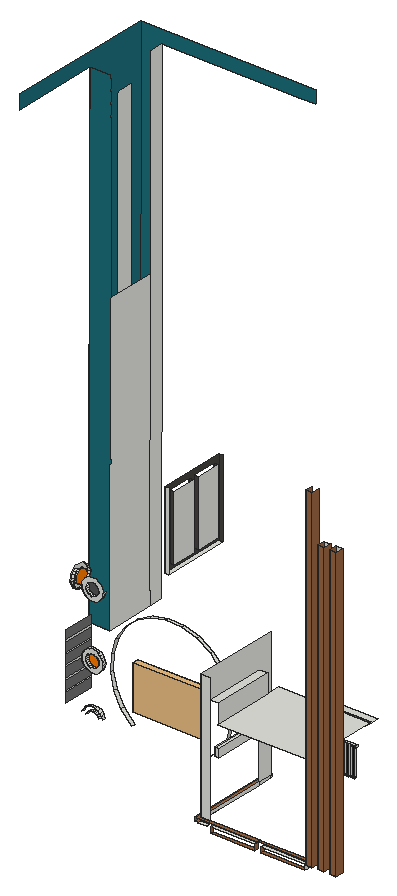
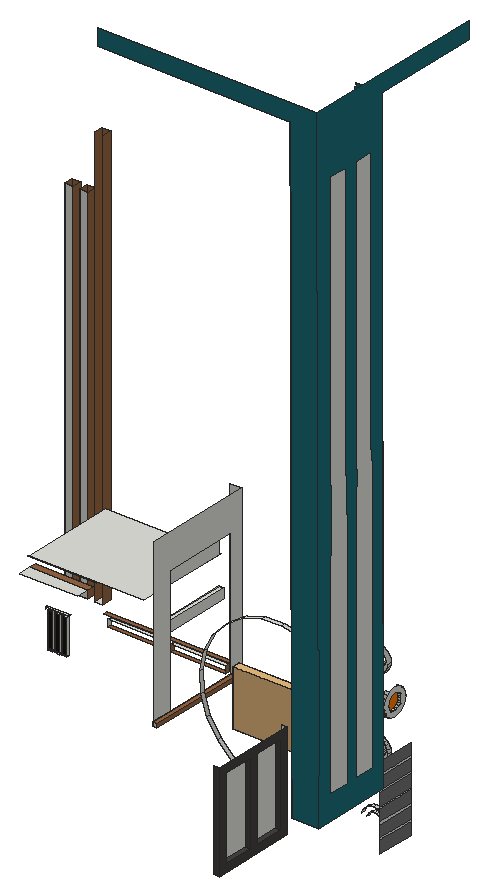
# SketchUp Ruby script. Lengths in inches.
U = 1.inch
M = Sketchup.active_model
def pt(a) = Geom::Point3d.new(a.map { |v| v * U })
def face(e, loops, mat)
  f = e.add_face(loops[0].map { |a| pt(a) })
  loops[1..].each { |l| e.add_face(l.map { |a| pt(a) }).erase! }
  f.material = f.back_material = mat if mat
  f
end
# faces: each face lists its corners as indices into pts; further lists are holes
def faces(e, pts, list, mat = nil) = list.each { |f| face(e, (f[0].is_a?(Array) ? f : [f]).map { |l| l.map { |i| pts[i] } }, mat) }
# xy, xz, yz: faces in a plane at the given z, y or x. An outline is a flat list of corners, or four numbers for a rectangle; further outlines are holes
def ring(l) = l.size == 4 ? [[l[0], l[1]], [l[2], l[1]], [l[2], l[3]], [l[0], l[3]]] : l.each_slice(2).to_a
def flat(e, list, mat, &to3) = list.each { |f| face(e, (f[0].is_a?(Array) ? f : [f]).map { |l| ring(l).map { |u, v| to3.(u, v) } }, mat) }
def xy(e, z, list, mat = nil) = flat(e, list, mat) { |x, y| [x, y, z] }
def xz(e, y, list, mat = nil) = flat(e, list, mat) { |x, z| [x, y, z] }
def yz(e, x, list, mat = nil) = flat(e, list, mat) { |y, z| [x, y, z] }
def lines(e, pts, list) = list.each { |a, b| e.add_line(pt(pts[a]), pt(pts[b])) }
# prism: a flat outline (further loops are holes) pulled along v
def prism(e, loops, v, mat = nil)
  f = face(e, loops, mat); d = Geom::Vector3d.new(v.map { |x| x * U })
  f.pushpull(f.normal.samedirection?(d) ? d.length : -d.length)
end
def box(e, o, s, mat = nil) = prism(e, [[o, [o[0] + s[0], o[1], o[2]], [o[0] + s[0], o[1] + s[1], o[2]], [o[0], o[1] + s[1], o[2]]]], [0, 0, s[2]], mat)
def at(x, y, z, deg = 0) = Geom::Transformation.translation(pt([x, y, z])) * Geom::Transformation.rotation(ORIGIN, Z_AXIS, deg.degrees)
def axes(o, x, y, z) = Geom::Transformation.new([*x, 0, *y, 0, *z, 0, *pt(o).to_a, 1])
def part(name) = M.definitions.add(name)
# library, detail: a bought-in or finely detailed component or shape, given as its bounding box
def library(name, o, s) = part(name).tap { |d| box(d.entities, o, s) }
def detail(e, o, s) = box(e.add_group.entities, o, s)
def put(e, d, t, mat = nil) = e.add_instance(d, t).tap { |i| i.material = mat if mat }
def group(e, t, mat = nil) = e.add_group.tap { |g| g.transformation = t; g.material = mat if mat }.entities
root = M.entities
M.materials.add("C05_Golden_Blaze").color = [255, 123, 0]
M.materials.add("I06_Sapphire_Night").color = [28, 110, 122]
M.materials.add("M05_Graphite_Haze").color = [114, 114, 114]
M.materials.add("M06_Steel_Smoke").color = [86, 86, 86]
M.materials.add("Wood_Floor_12_1K").color = [28, 22, 19]
M.materials.add("Wood_Planks_01_1K").color = [69, 67, 63]
M.materials.add("Wood_Veneer_15_1K").color = [153, 102, 66]
c1 = library("ALL HOUSE  DESIG",[0.14,0,0],[101.96,32.66,1])
box(root,[157.14,58,93.95],[2.5,40,5.23])
xy(root,54.33,[[161.64,48.875,190.64,50.875],[194.64,48.875,223.64,50.875]],"Wood_Veneer_15_1K")
xy(root,58,[[161.64,48.875,190.64,50.875],[194.64,48.875,223.64,50.875]])
xy(root,58,[[[151.11,48.875,151.11,109.2,153.64,109.2,153.64,50.875,159.64,50.875,159.64,48.875],[151.68,101.68,152.875,103],[151.68,93.68,152.875,95],[151.68,85.6875,152.875,87.01],[151.68,77.69,152.875,79.01],[151.68,69.7,152.875,71.02],[151.68,61.7,152.875,63.02]]],"Wood_Veneer_15_1K")
xy(root,58.02,[[153.64,48,159.64,50.875]])
xy(root,60,[[151.11,48.875,192.14,48.875,192.14,50.875,153.64,50.875,153.64,109.2,151.11,109.2],[193.14,48.875,225.64,50.875]],"Wood_Veneer_15_1K")
xy(root,61.78,[[228.57,43,232.92,48]])
xy(root,61.91,[[236.45,43,240.8,48]])
xy(root,62.04,[[244.33,43,248.68,48]])
xy(root,75.66,[[197.19,109.5,199.99,110.5],[200.99,109.5,203.79,110.5],[204.79,109.5,207.59,110.5]])
xy(root,76.43,[[197.19,109.5,199.99,110.5],[200.99,109.5,203.79,110.5],[204.79,109.5,207.59,110.5]])
xy(root,92.42,[[15.64,193.5,18.64,237.59]])
xy(root,94.34,[[197.19,109.5,199.99,110.5],[200.99,109.5,203.79,110.5],[204.79,109.5,207.59,110.5]])
xy(root,95.34,[[196.19,109.5,208.59,110.5]])
xy(root,96.42,[[15.64,197.5,18.64,213.54],[15.64,217.54,18.64,233.59]],"Wood_Planks_01_1K")
xy(root,111,[[186.64,110.5,216.64,117]])
xy(root,111,[[186.64,107,216.64,110.5]],"Wood_Veneer_15_1K")
xy(root,114,[[159.64,56.88,219.64,107]])
xy(root,114,[[183.64,107,219.64,108]],"Wood_Veneer_15_1K")
xy(root,126,[[[153.64,58,159.64,98],[158.35,92.29,158.94,95.07],[158.35,85.8,158.94,88.58],[158.35,79.31,158.94,82.09],[158.35,72.81,158.94,75.6],[158.35,66.32,158.94,69.11],[158.35,59.83,158.94,62.61]]])
xz(root,43,[[228.57,61.78,232.92,281.97],[236.45,61.91,240.8,252.41],[244.33,62.04,248.68,252.41]],"Wood_Veneer_15_1K")
xz(root,48,[[236.45,61.91,240.8,252.41],[244.33,62.04,248.68,252.41]])
xz(root,50.875,[[153.64,58,159.64,58.02],[153.64,58.02,159.64,60],[153.64,60,159.64,144]])
xz(root,106,[[[38.08,80.04,39.89,80.22,41.6,80.87,43.08,81.93,44.24,83.34,44.99,85,45.29,86.8,45.11,88.62,44.46,90.33,43.4,91.81,41.99,92.96,40.33,93.72,38.53,94.01,36.71,93.83,35,93.1875,33.52,92.125,32.37,90.71,31.61,89.05,31.32,87.25,31.5,85.4375,32.14,83.73,33.21,82.25,34.62,81.09,36.28,80.34],[38.3,82.78,37.2,82.93,36.18,83.35,35.3,84.03,34.625,84.91,34.2,85.93,34.06,87.03,34.2,88.125,34.625,89.15,35.3,90.03,36.18,90.7,37.2,91.13,38.3,91.27,39.4,91.13,40.43,90.7,41.3,90.03,41.98,89.15,42.4,88.125,42.55,87.03,42.4,85.93,41.98,84.91,41.3,84.03,40.43,83.35,39.4,82.93]],[[38.08,122.25,39.89,122.43,41.6,123.07,43.08,124.13,44.24,125.54,44.99,127.21,45.29,129.01,45.11,130.82,44.46,132.53,43.4,134.01,41.99,135.17,40.33,135.92,38.53,136.22,36.71,136.04,35,135.39,33.52,134.33,32.37,132.92,31.61,131.25,31.32,129.45,31.5,127.64,32.14,125.93,33.21,124.45,34.62,123.29,36.28,122.54],[38.17,124.95,37.0625,125.13,36.04,125.59,35.18,126.3,34.53,127.21,34.13,128.26,34.02,129.37,34.2,130.47,34.66,131.49,35.37,132.36,36.28,133.01,37.33,133.4,38.44,133.51,39.54,133.33,40.5625,132.87,41.43,132.16,42.08,131.25,42.47,130.21,42.58,129.09,42.4,127.99,41.94,126.97,41.23,126.11,40.32,125.45,39.28,125.06]]])
xz(root,108,[[38.3,82.78,39.4,82.93,40.43,83.35,41.3,84.03,41.98,84.91,42.4,85.93,42.55,87.03,42.4,88.125,41.98,89.15,41.3,90.03,40.43,90.7,39.4,91.13,38.3,91.27,37.2,91.13,36.18,90.7,35.3,90.03,34.625,89.15,34.2,88.125,34.06,87.03,34.2,85.93,34.625,84.91,35.3,84.03,36.18,83.35,37.2,82.93]],"C05_Golden_Blaze")
xz(root,108,[[38.17,124.95,39.28,125.06,40.32,125.45,41.23,126.11,41.94,126.97,42.4,127.99,42.58,129.09,42.47,130.21,42.08,131.25,41.43,132.16,40.5625,132.87,39.54,133.33,38.44,133.51,37.33,133.4,36.28,133.01,35.37,132.36,34.66,131.49,34.2,130.47,34.02,129.37,34.13,128.26,34.53,127.21,35.18,126.3,36.04,125.59,37.0625,125.13]],"M06_Steel_Smoke")
xz(root,109.2,[[151.11,58,153.64,60]])
xz(root,110.5,[[197.19,76.43,199.99,94.34],[200.99,76.43,203.79,94.34],[204.79,76.43,207.59,94.34]],"Wood_Floor_12_1K")
xz(root,134.17,[[27.27,88.73,27.64,284.16,27.64,284.36,27.82,380.13,27.84,390.13,26.84,390.13,26.84,392.13,27.84,392.13,27.85,397.81,26.85,397.81,26.86,399.81,27.86,399.81,27.87,405.49,26.87,405.49,26.875,407.49,27.875,407.49,27.88,413.16,26.88,413.17,26.89,415.17,13.74,415.19,13.12,88.76]],"I06_Sapphire_Night")
xz(root,176.1875,[[27.27,88.73,13.12,88.76,13.75,424.19,128.6,423.97,128.58,415.15,119.58,415.16,27.89,415.16,27.84,390.13,27.82,380.13,27.64,284.16]],"I06_Sapphire_Night")
xz(root,193.5,[[15.64,92.42,18.64,143.3]])
xz(root,197.5,[[15.64,96.42,18.64,139.3]],"Wood_Planks_01_1K")
xz(root,213.54,[[15.64,96.42,18.64,139.3]],"Wood_Planks_01_1K")
xz(root,217.54,[[15.64,96.42,18.64,139.3]],"Wood_Planks_01_1K")
xz(root,233.59,[[15.64,96.42,18.64,139.3]],"Wood_Planks_01_1K")
xz(root,237.59,[[15.64,92.42,18.64,143.3]],"Wood_Planks_01_1K")
yz(root,15.64,[[[193.5,92.42,237.59,143.3],[217.54,96.42,233.59,139.3],[197.5,96.42,213.54,139.3]]],"Wood_Planks_01_1K")
yz(root,16.64,[[[122.03,116,120.22,116.18,118.51,116.82,117.03,117.89,115.875,119.3,115.12,120.96,114.83,122.76,115.01,124.58,115.65,126.28,116.71,127.76,118.125,128.92,119.79,129.67,121.59,129.97,123.4,129.79,125.11,129.14,126.59,128.08,127.75,126.67,128.5,125.01,128.8,123.21,128.62,121.39,127.97,119.6875,126.91,118.2,125.5,117.05,123.83,116.3],[121.8125,118.74,122.91,118.88,123.93,119.31,124.8125,119.98,125.49,120.86,125.91,121.89,126.06,122.98,125.91,124.08,125.49,125.11,124.8125,125.99,123.93,126.66,122.91,127.08,121.8125,127.23,120.71,127.08,119.6875,126.66,118.81,125.99,118.13,125.11,117.71,124.08,117.57,122.98,117.71,121.89,118.13,120.86,118.81,119.98,119.6875,119.31,120.71,118.88]]])
yz(root,18.64,[[109,60.57,128.87,61.57],[109,68.01,128.87,69.01],[109,75.46,128.87,76.46],[109,82.9,128.87,83.9],[109,90.35,128.87,91.35],
  [197.5,96.42,213.54,139.3],[217.54,96.42,233.59,139.3]])
yz(root,18.64,[[121.8125,118.74,120.71,118.88,119.6875,119.31,118.81,119.98,118.13,120.86,117.71,121.89,117.57,122.98,117.71,124.08,118.13,125.11,118.81,125.99,119.6875,126.66,120.71,127.08,121.8125,127.23,122.91,127.08,123.93,126.66,124.8125,125.99,125.49,125.11,125.91,124.08,126.06,122.98,125.91,121.89,125.49,120.86,124.8125,119.98,123.93,119.31,122.91,118.88]],"C05_Golden_Blaze")
yz(root,18.64,[[109,54.12,128.87,60.57],[109,61.57,128.87,68.01],[109,69.01,128.87,75.46],[109,76.46,128.87,82.9],[109,83.9,128.87,90.35],
  [109,91.35,128.87,97.35]],"M05_Graphite_Haze")
yz(root,151.11,[[48.875,58,109.2,60]],"Wood_Veneer_15_1K")
yz(root,153.64,[[50.875,58,58,60],[58,58,98,60],[98,58,108,60],[108,58,109.2,60],[50.875,60,50.875,144,108,144,108,60,98,60,98,126,58,126,58,60]])
yz(root,159.64,[[48.875,58,50.875,58.02],[58,114,98,126]])
yz(root,161.64,[[48.875,54.33,50.875,58]],"Wood_Veneer_15_1K")
yz(root,190.64,[[48.875,54.33,50.875,58]],"Wood_Veneer_15_1K")
yz(root,194.64,[[48.875,54.33,50.875,58]],"Wood_Veneer_15_1K")
yz(root,197.19,[[109.5,76.43,110.5,94.34]])
yz(root,199.99,[[109.5,76.43,110.5,94.34]])
yz(root,200.99,[[109.5,76.43,110.5,94.34]])
yz(root,203.79,[[109.5,76.43,110.5,94.34]])
yz(root,204.79,[[109.5,76.43,110.5,94.34]])
yz(root,207.59,[[109.5,75.66,110.5,76.43],[109.5,76.43,110.5,94.34]])
yz(root,208.59,[[109.5,94.34,110.5,95.34]])
yz(root,223.64,[[48.875,54.33,50.875,58]])
yz(root,228.57,[[43,61.78,48,281.97]],"Wood_Veneer_15_1K")
yz(root,232.92,[[43,61.78,48,281.97]],"Wood_Veneer_15_1K")
yz(root,236.45,[[43,61.91,48,252.41]],"Wood_Veneer_15_1K")
yz(root,240.8,[[43,61.91,48,252.41]],"Wood_Veneer_15_1K")
yz(root,244.33,[[43,62.04,48,252.41]],"Wood_Veneer_15_1K")
yz(root,248.68,[[43,62.04,48,252.41]],"Wood_Veneer_15_1K")
p = [[34.2,108,54.32],[34.625,108,55.34],[34.625,106,55.34],[34.2,106,54.32],[41.98,108,55.34],[42.4,108,54.32],
  [42.4,106,54.32],[41.98,106,55.34],[45.11,108,54.81],[44.46,108,56.52],[44.46,106,56.52],[45.11,106,54.81],
  [32.37,108,56.9],[31.61,108,55.24],[31.61,106,55.24],[32.37,106,56.9],[35.3,108,56.22],[35.3,106,56.22],
  [41.3,108,56.22],[41.3,106,56.22],[112.8,108,55.62],[120.51,108,62.64],[120.51,106,62.64],[112.8,106,55.62],
  [36.18,108,56.89],[36.18,106,56.89],[40.43,108,56.89],[40.43,106,56.89],[43.4,108,58],[43.4,106,58],
  [33.52,108,58.32],[33.52,106,58.32],[37.2,108,57.32],[37.2,106,57.32],[39.4,108,57.32],[39.4,106,57.32],
  [38.3,108,57.46],[38.3,106,57.46],[57.2,108,65.59],[64.22,108,57.88],[64.22,106,57.88],[57.2,106,65.59],
  [41.99,108,59.15],[41.99,106,59.15],[35,108,59.38],[35,106,59.38],[40.33,108,59.91],[40.33,106,59.91],
  [36.71,108,60.02],[36.71,106,60.02],[38.53,108,60.2],[38.53,106,60.2],[126.14,108,71.42],[126.14,106,71.42],
  [52.42,108,74.86],[52.42,106,74.86],[129.3,108,81.35],[129.3,106,81.35],[50.19,108,85.04],[50.19,106,85.04],
  [36.28,108,80.34],[38.08,108,80.04],[38.08,106,80.04],[36.28,106,80.34],[39.89,108,80.22],[39.89,106,80.22],
  [41.6,108,80.87],[41.6,106,80.87],[34.62,108,81.09],[34.62,106,81.09],[43.08,108,81.93],[43.08,106,81.93],
  [33.21,108,82.25],[33.21,106,82.25],[129.79,108,91.77],[129.79,106,91.77],[44.24,108,83.34],[44.24,106,83.34],
  [32.14,108,83.73],[32.14,106,83.73],[38.3,108,82.78],[37.2,108,82.93],[37.2,106,82.93],[38.3,106,82.78],
  [39.4,108,82.93],[39.4,106,82.93],[36.18,108,83.35],[36.18,106,83.35],[40.43,108,83.35],[40.43,106,83.35],
  [44.99,108,85],[44.99,106,85],[35.3,108,84.03],[35.3,106,84.03],[41.3,108,84.03],[41.3,106,84.03],
  [31.5,108,85.4375],[31.5,106,85.4375],[34.625,108,84.91],[34.625,106,84.91],[41.98,108,84.91],[41.98,106,84.91],
  [34.2,108,85.93],[34.2,106,85.93],[42.4,108,85.93],[42.4,106,85.93],[45.29,108,86.8],[45.29,106,86.8],
  [50.68,108,95.46],[50.68,106,95.46],[31.32,108,87.25],[31.32,106,87.25],[34.06,108,87.03],[34.06,106,87.03],
  [42.55,108,87.03],[42.55,106,87.03],[45.11,108,88.62],[45.11,106,88.62],[34.2,108,88.125],[34.2,106,88.125],
  [42.4,108,88.125],[42.4,106,88.125],[31.61,108,89.05],[31.61,106,89.05],[34.625,108,89.15],[34.625,106,89.15],
  [41.98,108,89.15],[41.98,106,89.15],[44.46,108,90.33],[44.46,106,90.33],[27.27,167.15,88.73],[27.27,134.17,88.73],
  [13.12,134.17,88.76],[13.12,176.1875,88.76],[27.27,176.1875,88.73],[27.64,167.15,284.16],[27.64,134.17,284.16],[27.89,176.1875,415.16],
  [27.89,167.15,415.16],[27.84,167.15,390.13],[27.82,167.15,380.13],[27.64,167.15,284.36],[27.64,176.1875,284.16],[27.82,176.1875,380.13],
  [27.84,176.1875,390.13],[13.75,77.1875,424.19],[13.75,176.1875,424.19],[13.74,134.17,415.19],[13.74,77.1875,415.19],[13.69,157.68,390.5],
  [13.14,157.68,101.81],[13.14,167.91,101.81],[13.69,167.91,390.5],[13.14,140.9,101.81],[13.14,151.13,101.81],[13.69,151.13,390.5],
  [13.69,140.9,390.5],[32.37,108,90.71],[32.37,106,90.71],[35.3,108,90.03],[35.3,106,90.03],[41.3,108,90.03],
  [41.3,106,90.03],[36.18,108,90.7],[36.18,106,90.7],[40.43,108,90.7],[40.43,106,90.7],[43.4,108,91.81],
  [43.4,106,91.81],[33.52,108,92.125],[33.52,106,92.125],[37.2,108,91.13],[37.2,106,91.13],[39.4,108,91.13],
  [39.4,106,91.13],[38.3,108,91.27],[38.3,106,91.27],[41.99,108,92.96],[41.99,106,92.96],[127.5625,108,101.95],
  [127.5625,106,101.95],[35,108,93.1875],[35,106,93.1875],[40.33,108,93.72],[40.33,106,93.72],[36.71,108,93.83],
  [36.71,106,93.83],[38.53,108,94.01],[38.53,106,94.01],[53.84,108,105.39],[53.84,106,105.39],[122.78,108,111.21],
  [122.78,106,111.21],[59.47,108,114.17],[59.47,106,114.17],[115.75,108,118.92],[115.75,106,118.92],[67.18,108,121.19],
  [67.18,106,121.19],[18.64,122.03,116],[18.64,120.22,116.18],[16.64,120.22,116.18],[16.64,122.03,116],[18.64,123.83,116.3],
  [16.64,123.83,116.3],[18.64,118.51,116.82],[16.64,118.51,116.82],[18.64,125.5,117.05],[16.64,125.5,117.05],[18.64,117.03,117.89],
  [16.64,117.03,117.89],[18.64,126.91,118.2],[16.64,126.91,118.2],[18.64,115.875,119.3],[16.64,115.875,119.3],[18.64,127.97,119.6875],
  [16.64,127.97,119.6875],[18.64,120.71,118.88],[18.64,121.8125,118.74],[16.64,121.8125,118.74],[16.64,120.71,118.88],[18.64,122.91,118.88],
  [16.64,122.91,118.88],[106.98,108,124.55],[106.98,106,124.55],[18.64,119.6875,119.31],[16.64,119.6875,119.31],[18.64,123.93,119.31],
  [16.64,123.93,119.31],[18.64,115.12,120.96],[16.64,115.12,120.96],[18.64,118.81,119.98],[16.64,118.81,119.98],[18.64,124.8125,119.98],
  [16.64,124.8125,119.98],[18.64,128.62,121.39],[16.64,128.62,121.39],[18.64,118.13,120.86],[16.64,118.13,120.86],[18.64,125.49,120.86],
  [16.64,125.49,120.86],[18.64,117.71,121.89],[16.64,117.71,121.89],[18.64,125.91,121.89],[16.64,125.91,121.89],[18.64,114.83,122.76],
  [16.64,114.83,122.76],[76.44,108,125.98],[76.44,106,125.98],[18.64,128.8,123.21],[16.64,128.8,123.21],[18.64,117.57,122.98],
  [16.64,117.57,122.98],[18.64,126.06,122.98],[16.64,126.06,122.98],[36.28,108,122.54],[38.08,108,122.25],[38.08,106,122.25],
  [36.28,106,122.54],[39.89,108,122.43],[39.89,106,122.43],[41.6,108,123.07],[41.6,106,123.07],[34.62,108,123.29],
  [34.62,106,123.29],[18.64,115.01,124.58],[16.64,115.01,124.58],[18.64,117.71,124.08],[16.64,117.71,124.08],[18.64,125.91,124.08],
  [16.64,125.91,124.08],[43.08,108,124.13],[43.08,106,124.13],[18.64,128.5,125.01],[16.64,128.5,125.01],[33.21,108,124.45],
  [33.21,106,124.45],[44.24,108,125.54],[44.24,106,125.54],[18.64,118.13,125.11],[16.64,118.13,125.11],[18.64,125.49,125.11],
  [16.64,125.49,125.11],[32.14,108,125.93],[32.14,106,125.93],[97.04,108,127.72],[97.04,106,127.72],[18.64,115.65,126.28],
  [16.64,115.65,126.28],[38.17,108,124.95],[37.0625,108,125.13],[37.0625,106,125.13],[38.17,106,124.95],[39.28,108,125.06],
  [39.28,106,125.06],[18.64,127.75,126.67],[16.64,127.75,126.67],[36.04,108,125.59],[36.04,106,125.59],[40.32,108,125.45],
  [40.32,106,125.45],[18.64,118.81,125.99],[16.64,118.81,125.99],[18.64,124.8125,125.99],[16.64,124.8125,125.99],[41.23,108,126.11],
  [41.23,106,126.11],[44.99,108,127.21],[44.99,106,127.21],[35.18,108,126.3],[35.18,106,126.3],[31.5,108,127.64],
  [31.5,106,127.64],[86.63,108,128.2],[86.63,106,128.2],[18.64,119.6875,126.66],[16.64,119.6875,126.66],[18.64,123.93,126.66],
  [16.64,123.93,126.66],[41.94,108,126.97],[41.94,106,126.97],[34.53,108,127.21],[34.53,106,127.21],[18.64,116.71,127.76],
  [16.64,116.71,127.76],[18.64,120.71,127.08],[16.64,120.71,127.08],[18.64,122.91,127.08],[16.64,122.91,127.08],[18.64,126.59,128.08],
  [16.64,126.59,128.08],[42.4,108,127.99],[42.4,106,127.99],[18.64,121.8125,127.23],[16.64,121.8125,127.23],[34.13,108,128.26],
  [34.13,106,128.26],[45.29,108,129.01],[45.29,106,129.01],[31.32,108,129.45],[31.32,106,129.45],[18.64,118.125,128.92],
  [16.64,118.125,128.92],[42.58,108,129.09],[42.58,106,129.09],[18.64,125.11,129.14],[16.64,125.11,129.14],[34.02,108,129.37],
  [34.02,106,129.37],[199.99,110.5,75.66],[199.99,110.5,76.43],[203.79,110.5,75.66],[203.79,110.5,76.43],[38.3,108,124.99],
  [37.2,108,125.13],[36.18,108,125.55],[35.3,108,126.23],[34.625,108,127.11],[34.2,108,128.13],[34.06,108,129.23],
  [42.55,108,129.23],[42.4,108,128.13],[41.98,108,127.11],[41.3,108,126.23],[40.43,108,125.55],[39.4,108,125.13]]
faces(root,p,[[0,1,2,3],[4,5,6,7],[8,9,10,11],[12,13,14,15],[1,16,17,2],[18,4,7,19],[20,21,22,23],[16,24,25,17],
  [26,18,19,27],[9,28,29,10],[30,12,15,31],[24,32,33,25],[34,26,27,35],[32,36,37,33],[36,34,35,37],[38,39,40,41],
  [28,42,43,29],[44,30,31,45],[42,46,47,43],[48,44,45,49],[46,50,51,47],[50,48,49,51],[21,52,53,22],[54,38,41,55],
  [52,56,57,53],[58,54,55,59],[60,61,62,63],[61,64,65,62],[64,66,67,65],[68,60,63,69],[66,70,71,67],[72,68,69,73],
  [56,74,75,57],[70,76,77,71],[78,72,73,79],[80,81,82,83],[84,80,83,85],[81,86,87,82],[88,84,85,89],[76,90,91,77],
  [86,92,93,87],[94,88,89,95],[96,78,79,97],[92,98,99,93],[100,94,95,101],[98,102,103,99],[104,100,101,105],[90,106,107,91],
  [108,58,59,109],[110,96,97,111],[102,112,113,103],[114,104,105,115],[106,116,117,107],[112,118,119,113],[120,114,115,121],[122,110,111,123],
  [118,124,125,119],[126,120,121,127],[116,128,129,117],[130,131,132,133,134],[130,135,136,131],[137,138,139,140,141,135,130,134,142,143,144],[157,122,123,158],[124,159,160,125],
  [161,126,127,162],[159,163,164,160],[165,161,162,166],[128,167,168,129],[169,157,158,170],[163,171,172,164],[173,165,166,174],[171,175,176,172],
  [175,173,174,176],[167,177,178,168],[74,179,180,75],[181,169,170,182],[177,183,184,178],[185,181,182,186],[183,187,188,184],[187,185,186,188],
  [189,108,109,190],[154,153,156,155],[150,149,152,151],[179,191,192,180],[193,189,190,194],[191,195,196,192],[197,193,194,198],[199,200,201,202],
  [203,199,202,204],[200,205,206,201],[207,203,204,208],[205,209,210,206],[211,207,208,212],[209,213,214,210],[215,211,212,216],[217,218,219,220],
  [218,221,222,219],[195,223,224,196],[225,217,220,226],[221,227,228,222],[213,229,230,214],[231,225,226,232],[227,233,234,228],[235,215,216,236],
  [237,231,232,238],[233,239,240,234],[241,237,238,242],[239,243,244,240],[229,245,246,230],[247,197,198,248],[249,235,236,250],[251,241,242,252],
  [243,253,254,244],[255,256,257,258],[256,259,260,257],[259,261,262,260],[263,255,258,264],[245,265,266,246],[267,251,252,268],[253,269,270,254],
  [261,271,272,262],[273,249,250,274],[275,263,264,276],[271,277,278,272],[279,267,268,280],[269,281,282,270],[283,275,276,284],[223,285,286,224],
  [265,287,288,266],[289,290,291,292],[293,289,292,294],[295,273,274,296],[290,297,298,291],[299,293,294,300],[301,279,280,302],[281,303,304,282],
  [305,299,300,306],[277,307,308,278],[297,309,310,298],[311,283,284,312],[313,247,248,314],[315,301,302,316],[303,317,318,304],[319,305,306,320],
  [309,321,322,310],[287,323,324,288],[325,315,316,326],[317,327,328,318],[329,295,296,330],[331,319,320,332],[333,325,326,334],[327,333,334,328],
  [321,335,336,322],[307,337,338,308],[339,311,312,340],[285,313,314,286],[323,341,342,324],[343,331,332,344],[345,329,330,346],[335,347,348,336]])
faces(root,p,[[[145,146,133,132,147,148],[149,150,151,152],[153,154,155,156]]],"I06_Sapphire_Night")
lines(root,p,[[349,350],[351,352],[353,354],[354,355],[355,356],[356,357],[357,358],[358,359],[360,361],[361,362],[362,363],[363,364],
  [364,365],[365,353]])
put(root,c1,axes([68.02,106,69.41],[0.4522,0,0],[0,0,0.89],[0,-4.2978,0]))
